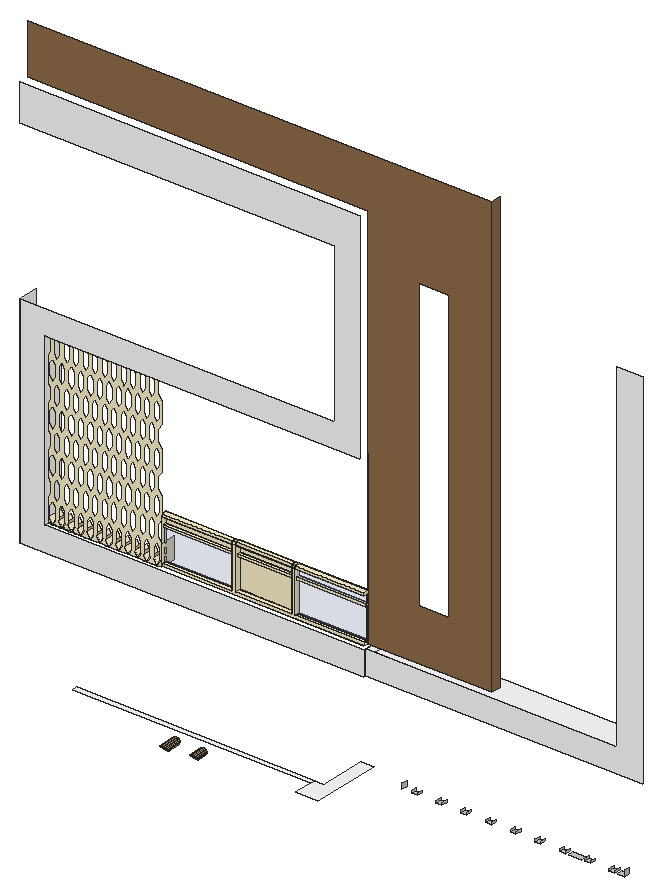
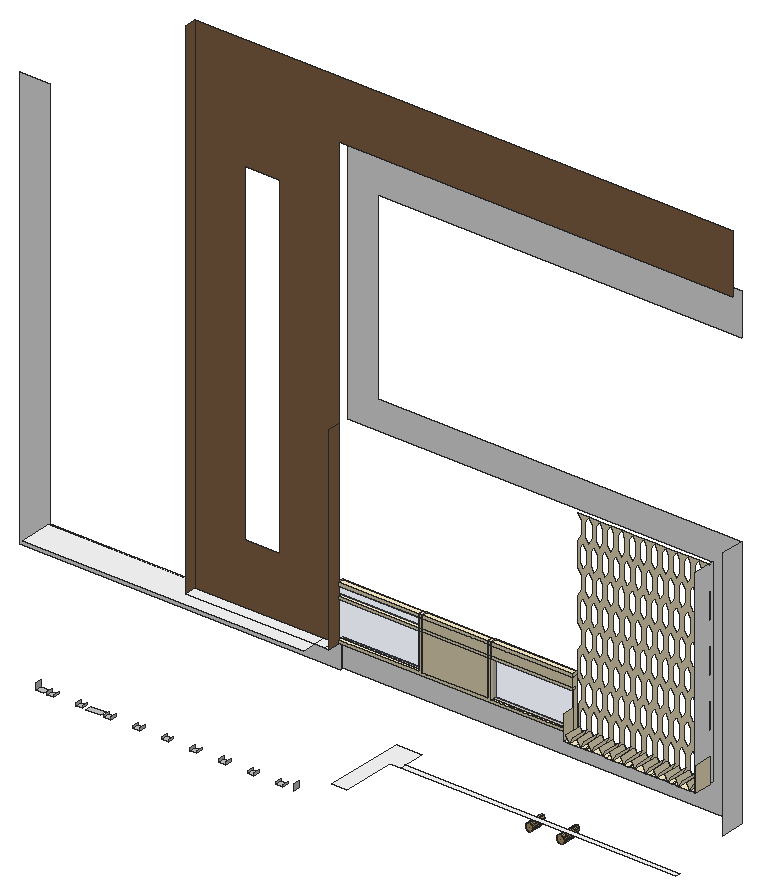
# SketchUp Ruby script. Lengths in inches.
U = 1.inch
M = Sketchup.active_model
def pt(a) = Geom::Point3d.new(a.map { |v| v * U })
def face(e, loops, mat)
  f = e.add_face(loops[0].map { |a| pt(a) })
  loops[1..].each { |l| e.add_face(l.map { |a| pt(a) }).erase! }
  f.material = f.back_material = mat if mat
  f
end
# faces: each face lists its corners as indices into pts; further lists are holes
def faces(e, pts, list, mat = nil) = list.each { |f| face(e, (f[0].is_a?(Array) ? f : [f]).map { |l| l.map { |i| pts[i] } }, mat) }
# xy, xz, yz: faces in a plane at the given z, y or x. An outline is a flat list of corners, or four numbers for a rectangle; further outlines are holes
def ring(l) = l.size == 4 ? [[l[0], l[1]], [l[2], l[1]], [l[2], l[3]], [l[0], l[3]]] : l.each_slice(2).to_a
def flat(e, list, mat, &to3) = list.each { |f| face(e, (f[0].is_a?(Array) ? f : [f]).map { |l| ring(l).map { |u, v| to3.(u, v) } }, mat) }
def xy(e, z, list, mat = nil) = flat(e, list, mat) { |x, y| [x, y, z] }
def xz(e, y, list, mat = nil) = flat(e, list, mat) { |x, z| [x, y, z] }
def yz(e, x, list, mat = nil) = flat(e, list, mat) { |y, z| [x, y, z] }
def lines(e, pts, list) = list.each { |a, b| e.add_line(pt(pts[a]), pt(pts[b])) }
# prism: a flat outline (further loops are holes) pulled along v
def prism(e, loops, v, mat = nil)
  f = face(e, loops, mat); d = Geom::Vector3d.new(v.map { |x| x * U })
  f.pushpull(f.normal.samedirection?(d) ? d.length : -d.length)
end
def box(e, o, s, mat = nil) = prism(e, [[o, [o[0] + s[0], o[1], o[2]], [o[0] + s[0], o[1] + s[1], o[2]], [o[0], o[1] + s[1], o[2]]]], [0, 0, s[2]], mat)
def at(x, y, z, deg = 0) = Geom::Transformation.translation(pt([x, y, z])) * Geom::Transformation.rotation(ORIGIN, Z_AXIS, deg.degrees)
def axes(o, x, y, z) = Geom::Transformation.new([*x, 0, *y, 0, *z, 0, *pt(o).to_a, 1])
def part(name) = M.definitions.add(name)
# library, detail: a bought-in or finely detailed component or shape, given as its bounding box
def library(name, o, s) = part(name).tap { |d| box(d.entities, o, s) }
def detail(e, o, s) = box(e.add_group.entities, o, s)
def put(e, d, t, mat = nil) = e.add_instance(d, t).tap { |i| i.material = mat if mat }
def group(e, t, mat = nil) = e.add_group.tap { |g| g.transformation = t; g.material = mat if mat }.entities
root = M.entities
M.materials.add("D01_Frost_White").color = [255, 242, 206]
M.materials.add("Glass_Sky Reflection_01").color = [126, 138, 183]
M.materials["Glass_Sky Reflection_01"].alpha = 0.25
M.materials.add("M00_Soft_Cloud").color = [255, 255, 255]
M.materials.add("Metal_Perforated_03_1K").color = [205, 205, 205]
M.materials.add("Plywood_08_1K").color = [202, 166, 113]
M.materials.add("Wood_Floor_01_1K").color = [146, 111, 76]
xy(root,51.6968,[[394.8388,115.4372,398.9652,119.1663],[412.2906,115.4372,416.417,119.1663],[429.7424,115.4372,433.8688,119.1663],[447.1942,115.4372,451.3206,119.1663],[464.646,115.4372,468.7724,119.1663],
  [482.0978,115.4372,486.2242,119.1663],[499.5496,115.4372,503.676,119.1663],[517.0014,115.4372,521.1278,119.1663],[534.4532,115.4372,538.5796,119.1663]],"Metal_Perforated_03_1K")
xy(root,51.7981,[[505.7245,115.4372,514.9529,119.1663],[540.6281,115.4372,545.2423,119.1663]],"Metal_Perforated_03_1K")
xy(root,60,[[353.5364,64.7712,369.0099,64.7712,369.0099,114,360.228,114,360.228,81.2712,353.5364,81.2712],[185.5364,78.2712,353.5364,81.2712]],"M00_Soft_Cloud")
xy(root,137.0192,[[209.933,109.0676,210.1614,119.6039],[210.1614,109.0676,211.0379,119.6039],[211.0379,109.0676,213.2784,119.6039],[213.2784,109.0676,216.6239,119.6039],[216.6239,109.0676,219.9694,119.6039],
  [219.9694,109.0676,223.3148,119.6039]],"D01_Frost_White")
xy(root,137.0192,[[368.5859,108.0124,368.7779,112.9098],[368.7779,108.0124,375,112.9098],[375,108.0124,546,108.0124,546,128.0311,375,128.0311,375,120,453.2434,120,453.2434,112.9098,375,112.9098],[366,112.9098,368.5859,120],[368.5859,112.9098,368.7779,120],
  [368.7779,112.9098,375,120],[368.7779,112.9098,375,120],[375,112.9098,453.2434,120]],"M00_Soft_Cloud")
xy(root,137.0253,[[183.1692,109.0676,183.3976,119.6039],[183.3976,109.0676,184.2742,119.6039],[184.2742,109.0676,186.5147,119.6039],[186.5147,109.0676,189.8602,119.6039],[189.8602,109.0676,193.2056,119.6039],
  [193.2056,109.0676,197.6561,119.6039],[197.6561,109.0676,199.8966,119.6039],[199.8966,109.0676,206.5875,119.6039],[206.5875,109.0676,209.933,119.6039]],"D01_Frost_White")
xy(root,137.0314,[[156.4055,109.0676,156.6339,119.6039],[156.6339,109.0676,157.5105,119.6039],[157.5105,109.0676,159.751,119.6039],[159.751,109.0676,163.0964,119.6039],[163.0964,109.0676,166.4419,119.6039],
  [166.4419,109.0676,169.7874,119.6039],[169.7874,109.0676,170.0158,119.6039],[170.0158,109.0676,170.8923,119.6039],[170.8923,109.0676,173.1328,119.6039],[173.1328,109.0676,179.8238,119.6039],
  [179.8238,109.0676,183.1692,119.6039]],"D01_Frost_White")
xy(root,137.0374,[[143.0236,109.0676,143.252,119.6039],[143.252,109.0676,144.1286,119.6039],[144.1286,109.0676,146.3691,119.6039],[146.3691,109.0676,153.06,119.6039],[153.06,109.0676,156.4055,119.6039]],"D01_Frost_White")
xy(root,137.5531,[[223.3148,109.5873,366.1463,113.1759]],"D01_Frost_White")
xy(root,139.4984,[[223.3148,109.5873,272.8822,111.884],[275.1001,109.5873,314.9232,113.1759],[317.1411,109.5873,366.1463,111.3816],[317.1411,111.3816,366.1463,113.1759],[223.3148,111.884,272.8822,113.1759]],"D01_Frost_White")
xy(root,161.637,[[223.3148,110.5921,366.1463,113.1759]],"D01_Frost_White")
xy(root,163.1544,[[223.3148,110.5921,366.1463,113.1759]],"D01_Frost_White")
xy(root,168.938,[[223.3148,109.5873,366.1463,113.1759]],"D01_Frost_White")
xy(root,170.8834,[[223.3148,109.5873,272.8822,113.1759],[272.8822,109.5873,275.1001,113.1759],[275.1001,109.5873,314.9232,113.1759],[314.9232,109.5873,317.1411,113.1759],[317.1411,109.5873,366.1463,113.1759]],"D01_Frost_White")
xz(root,78.2712,[[258.3445,50.6009,257.7234,50.6827,257.1447,50.9224,256.6477,51.3038,256.2664,51.8007,256.0266,52.3795,255.9449,53.0005,256.0266,53.6216,256.2664,54.2003,256.6477,54.6973,257.1447,55.0786,257.7234,55.3184,258.3445,55.4001,258.9655,55.3184,259.5443,55.0786,260.0412,54.6973,260.4226,54.2003,260.6623,53.6216,260.7441,53.0005,260.6623,52.3795,260.4226,51.8007,260.0412,51.3038,259.5443,50.9224,258.9655,50.6827],[277.4723,50.6009,276.8512,50.6827,276.2725,50.9224,275.7755,51.3038,275.3941,51.8007,275.1544,52.3795,275.0727,53.0005,275.1544,53.6216,275.3941,54.2003,275.7755,54.6973,276.2725,55.0786,276.8512,55.3184,277.4723,55.4001,278.0933,55.3184,278.6721,55.0786,279.169,54.6973,279.5504,54.2003,279.7901,53.6216,279.8719,53.0005,279.7901,52.3795,279.5504,51.8007,279.169,51.3038,278.6721,50.9224,278.0933,50.6827]],"Plywood_08_1K")
xz(root,105.8195,[[126,120,368.7779,120,368.7779,137.0192,143.4397,137.0192,143.4397,257.0192,366,257.0192,366,411.0577,126,411.0577,126,385.4776,348,385.4776,348,274.0384,126,274.0384]],"M00_Soft_Cloud")
xz(root,108.0124,[[368.5859,119.9631,564,119.9631,564,377.4389,546,377.4389,546,137.0192,368.5859,137.0192]],"M00_Soft_Cloud")
xz(root,109.0676,[[[209.933,137.0192,213.2784,137.0192,211.0744,140.7687,211.0744,148.2675,213.2784,152.0169,215.4825,148.2675,215.4825,140.7687,213.2784,137.0192,219.9694,137.0192,217.7653,140.7687,217.7653,148.2675,219.9694,152.0169,222.1734,148.2675,222.1734,140.7687,219.9694,137.0192,223.3148,137.0192,223.3148,152.0169,221.1108,155.7664,221.1108,163.2652,223.3148,167.0147,223.3148,182.0124,221.1108,185.7618,221.1108,193.2607,223.3148,197.0101,223.3077,197.0101,223.3077,212.0078,221.1037,215.7573,221.1037,223.2561,223.3077,227.0056,223.3077,242.0033,221.1037,245.7527,221.1037,253.2516,223.3077,257.001,216.6168,257.001,218.8208,253.2516,218.8208,245.7527,216.6168,242.0033,214.4127,245.7527,214.4127,253.2516,216.6168,257.001,209.933,257.001,209.933,256.9889,212.1299,253.2516,212.1299,245.7527,209.933,242.0154,209.933,242.0094,209.9312,242.0124,207.7289,245.7588,207.7289,253.2576,209.9276,256.998,209.9258,257.001,209.9294,257.001,209.933,257.0071,203.242,257.0071,205.4461,253.2576,205.4461,245.7588,203.242,242.0094,201.038,245.7588,201.038,253.2576,203.242,257.0071,196.5511,257.0071,196.5529,257.004,196.5547,257.004,196.5547,257.001,198.7552,253.2576,198.7552,245.7588,198.7444,245.7406,198.7409,245.7345,198.7337,245.7225,196.5404,242.0154,196.5368,242.0094,196.5261,242.0276,195.4366,243.8932,195.801,243.2733,194.3399,245.783,194.3399,245.7709,194.3363,245.777,194.3364,245.7891,194.3363,245.7892,194.3364,245.8134,194.3399,249.5264,194.3399,248.2868,194.347,253.2698,194.3542,253.2819,195.0829,254.5216,195.4473,255.1415,196.5422,257.004,189.8548,257.004,192.0571,253.2576,192.0571,245.7588,189.853,242.0094,187.649,245.7588,187.649,253.2576,189.8512,257.004,183.1639,257.004,185.3661,253.2576,185.3661,245.7588,183.1675,242.0185,183.1639,242.0124,183.1639,242.0245,180.9652,245.7649,180.9652,253.2637,183.1639,257.004,183.1621,257.0071,183.1657,257.0071,183.1692,257.0132,176.4783,257.0132,178.6824,253.2637,178.6824,245.7649,176.4783,242.0154,174.2743,245.7649,174.2743,253.2637,176.4783,257.0132,169.7874,257.0132,171.9878,253.2576,171.9843,245.7649,169.7802,242.0276,167.5797,245.7709,167.5797,253.2698,167.5833,253.2759,169.7838,257.0192,163.0929,257.0192,165.2969,253.2698,165.2969,245.7709,163.0929,242.0215,160.8888,245.7709,160.8888,253.2698,163.0929,257.0192,156.4055,257.0192,156.4037,257.0162,158.606,253.2698,158.606,245.7709,156.4037,242.0245,154.2015,245.7709,154.2015,253.2698,156.4037,257.0162,156.4019,257.0192,149.7146,257.0192,151.9186,253.2698,151.9186,245.7709,149.7146,242.0215,147.5105,245.7709,147.5105,253.2698,149.7146,257.0192,143.0236,257.0192,145.2277,253.2698,145.2277,245.7709,143.0236,242.0215,143.0236,227.0238,145.2277,223.2743,145.2277,215.7755,143.0236,212.0261,143.0236,197.0283,143.0271,197.0224,143.0272,197.0223,145.2277,193.2789,145.2277,185.78,143.0236,182.0306,143.0236,167.0329,145.2277,163.2835,145.2277,155.7846,143.0236,152.0352,143.0236,137.0374,146.3691,137.0374,144.165,140.7869,144.165,148.2857,146.3691,152.0352,148.5731,148.2857,148.5731,140.7869,146.3691,137.0374,153.06,137.0374,150.856,140.7869,150.856,148.2857,153.06,152.0352,155.2641,148.2857,155.2641,140.7869,153.06,137.0374,156.4055,137.0374,156.4055,137.0314,159.751,137.0314,157.5469,140.7808,157.5469,148.2797,159.751,152.0291,161.955,148.2797,161.955,140.7808,159.751,137.0314,166.4419,137.0314,164.2379,140.7808,164.2379,148.2797,166.4419,152.0291,168.6459,148.2797,168.6459,140.7808,166.4419,137.0314,173.1328,137.0314,170.9288,140.7808,170.9288,148.2797,173.1328,152.0291,175.3369,148.2797,175.3369,140.7808,173.1328,137.0314,179.8238,137.0314,177.6197,140.7808,177.6197,148.2797,179.8238,152.0291,182.0278,148.2797,182.0278,140.7808,179.8238,137.0314,183.1692,137.0314,183.1692,137.0253,186.5147,137.0253,184.3107,140.7747,184.3107,148.2736,186.5147,152.023,188.7188,148.2736,188.7188,140.7747,186.5147,137.0253,193.2056,137.0253,191.0016,140.7747,191.0016,148.2736,193.2056,152.023,195.4097,148.2736,195.4097,140.7747,193.2056,137.0253,199.8966,137.0253,197.6925,140.7747,197.6925,148.2736,199.8966,152.023,202.1006,148.2736,202.1006,140.7747,199.8966,137.0253,206.5875,137.0253,204.3835,140.7747,204.3835,148.2736,206.5875,152.023,208.7916,148.2736,208.7916,140.7747,206.5875,137.0253,209.933,137.0253],[169.7874,182.0245,168.6907,183.8901,167.5869,185.7557,167.5869,185.7679,167.5833,185.774,167.5833,189.5052,167.5797,193.2546,167.5833,193.2607,167.5833,193.2728,168.68,195.1384,169.7802,197.0223,169.7874,197.0223,169.7909,197.0163,169.7909,197.0162,170.884,195.1567,171.9878,193.2911,171.9879,193.2789,171.9914,193.2728,171.9914,189.5416,171.995,185.7922,171.9914,185.7861,171.9914,185.774,170.8947,183.9084,169.7945,182.0245,169.7909,182.0306],[189.8602,182.0185,187.6561,185.7679,187.6561,193.2668,189.8566,197.0101,189.8495,197.0101,189.8514,197.0134,189.853,197.0162,189.8602,197.0162,189.8637,197.0101,192.0642,193.2668,192.0642,185.7679],[196.5511,182.0185,194.3471,185.7679,194.3471,193.2668,196.5475,197.0101,196.5404,197.0101,196.544,197.0162,196.5511,197.0162,196.5546,197.0102,196.5547,197.0101,198.7552,193.2668,198.7552,185.7679],[216.6239,182.0124,214.4199,185.7618,214.4199,193.2607,216.6203,197.004,216.6184,197.0073,216.6168,197.0101,216.6239,197.0101,218.828,193.2607,218.828,185.7618],[163.0964,182.0245,160.8924,185.774,160.8924,193.2728,163.0964,197.0223,163.0893,197.0223,163.0912,197.0256,163.0929,197.0283,163.0945,197.0256,163.0964,197.0223,165.3005,193.2728,165.3005,185.774],[209.933,182.0124,209.933,182.0185,207.7289,185.7679,207.7289,193.2668,209.9276,197.0071,209.9258,197.0101,209.9294,197.0101,209.933,197.0162,209.933,197.0101,212.137,193.2607,212.137,185.7618],[203.242,212.0139,201.038,215.7633,201.038,223.2622,203.242,227.0116,205.4461,223.2622,205.4461,215.7633],[163.0929,212.0261,160.8888,215.7755,160.8888,223.2743,163.0929,227.0238,165.2969,223.2743,165.2969,215.7755],[189.853,212.0139,187.649,215.7633,187.649,223.2622,189.853,227.0116,192.0571,223.2622,192.0571,215.7633],[216.6168,212.0078,214.4127,215.7573,214.4127,223.2561,216.6168,227.0056,218.8208,223.2561,218.8208,215.7573],[196.544,212.0139,194.3399,215.7633,194.3399,223.2622,196.544,227.0116,198.748,223.2622,198.748,215.7633],[206.5875,197.0162,204.3835,200.7656,204.3835,208.2645,206.5875,212.0139,208.7916,208.2645,208.7916,200.7656],[199.8966,197.0162,197.6925,200.7656,197.6925,208.2645,199.8966,212.0139,202.1006,208.2645,202.1006,200.7656],[186.5076,197.0162,184.3035,200.7656,184.3035,208.2645,186.5076,212.0139,188.7116,208.2645,188.7116,200.7656],[166.4383,197.0283,164.2343,200.7778,164.2343,208.2766,166.4383,212.0261,168.6424,208.2766,168.6424,200.7778],[159.7474,197.0283,157.5433,200.7778,157.5433,208.2766,159.7474,212.0261,161.9514,208.2766,161.9514,200.7778],[193.1985,197.0162,190.9945,200.7656,190.9945,208.2645,193.1985,212.0139,195.4025,208.2645,195.4025,200.7656],[219.9622,197.0101,217.7582,200.7595,217.7582,208.2584,219.9622,212.0078,222.1663,208.2584,222.1663,200.7595],[213.2713,197.0101,211.0673,200.7595,211.0673,208.2584,213.2713,212.0078,215.4754,208.2584,215.4754,200.7595],[189.8602,152.023,187.6561,155.7725,187.6561,163.2713,189.8602,167.0207,192.0642,163.2713,192.0642,155.7725],[176.4783,212.02,174.2743,215.7694,174.2743,223.2683,176.4783,227.0177,178.6824,223.2683,178.6824,215.7694],[156.4055,182.0245,156.4055,182.0306,154.2015,185.78,154.2015,193.2789,156.4019,197.0223,156.4055,197.0283,156.4055,197.0223,158.6095,193.2728,158.6095,185.774],[149.7146,212.0261,147.5105,215.7755,147.5105,223.2743,149.7146,227.0238,151.9186,223.2743,151.9186,215.7755],[163.0964,152.0291,160.8924,155.7785,160.8924,163.2774,163.0964,167.0268,165.3005,163.2774,165.3005,155.7785],[176.4783,182.0245,174.2743,185.774,174.2743,193.2728,176.4747,197.0162,176.4767,197.0195,176.4783,197.0223,176.4799,197.0195,176.4819,197.0162,178.6824,193.2728,178.6824,185.774],[149.7146,152.0352,147.5105,155.7846,147.5105,163.2835,149.7146,167.0329,151.9186,163.2835,151.9186,155.7846],[156.4055,152.0291,156.4055,152.0352,154.2015,155.7846,154.2015,163.2835,156.4055,167.0329,156.4055,167.0268,158.6095,163.2774,158.6095,155.7785],[149.7146,182.0306,147.5105,185.78,147.5105,193.2789,149.711,197.0223,149.7129,197.0256,149.7146,197.0283,149.7162,197.0256,149.7181,197.0223,151.9186,193.2789,151.9186,185.78],[169.7874,152.0291,167.5833,155.7785,167.5833,163.2774,169.7874,167.0268,171.9914,163.2774,171.9914,155.7785],[183.1692,152.023,183.1692,152.0291,180.9652,155.7785,180.9652,163.2774,183.1692,167.0268,183.1692,167.0207,185.3733,163.2713,185.3733,155.7725],[179.8238,197.0223,177.6197,200.7717,177.6197,208.2706,179.8238,212.02,182.0278,208.2706,182.0278,200.7717],[173.1328,197.0223,170.9288,200.7717,170.9288,208.2706,173.1328,212.02,175.3369,208.2706,175.3369,200.7717],[146.3691,197.0283,144.165,200.7778,144.165,208.2766,146.3691,212.0261,148.5731,208.2766,148.5731,200.7778],[153.06,197.0283,150.856,200.7778,150.856,208.2766,153.06,212.0261,155.2641,208.2766,155.2641,200.7778],[196.5511,152.023,194.3471,155.7725,194.3471,163.2713,196.5511,167.0207,198.7552,163.2713,198.7552,155.7725],[176.4783,152.0291,174.2743,155.7785,174.2743,163.2774,176.4783,167.0268,178.6824,163.2774,178.6824,155.7785],[179.8238,167.0268,177.6197,170.7762,177.6197,178.2751,179.8238,182.0245,182.0278,178.2751,182.0278,170.7762],[216.6239,152.0169,214.4199,155.7664,214.4199,163.2652,216.6239,167.0147,218.828,163.2652,218.828,155.7664],[173.1328,167.0268,170.9288,170.7762,170.9288,178.2751,173.1328,182.0245,175.3369,178.2751,175.3369,170.7762],[153.06,167.0329,150.856,170.7823,150.856,178.2812,153.06,182.0306,155.2641,178.2812,155.2641,170.7823],[209.933,152.0169,209.933,152.023,207.7289,155.7725,207.7289,163.2713,209.933,167.0207,209.933,167.0147,212.137,163.2652,212.137,155.7664],[146.3691,167.0329,144.165,170.7823,144.165,178.2812,146.3691,182.0306,148.5731,178.2812,148.5731,170.7823],[186.5147,167.0207,184.3107,170.7702,184.3107,178.269,186.5147,182.0185,188.7188,178.269,188.7188,170.7702],[193.2056,167.0207,191.0016,170.7702,191.0016,178.269,193.2056,182.0185,195.4097,178.269,195.4097,170.7702],[173.1328,227.0177,170.9288,230.7671,170.9288,238.266,173.1328,242.0154,175.3369,238.266,175.3369,230.7671],[179.8238,227.0177,177.6197,230.7671,177.6197,238.266,179.8238,242.0154,182.0278,238.266,182.0278,230.7671],[166.4419,167.0268,164.2379,170.7762,164.2379,178.2751,166.4419,182.0245,168.6459,178.2751,168.6459,170.7762],[159.751,167.0268,157.5469,170.7762,157.5469,178.2751,159.751,182.0245,161.955,178.2751,161.955,170.7762],[203.242,182.0185,201.038,185.7679,201.038,193.2668,203.2385,197.0101,203.2404,197.0134,203.242,197.0162,203.2437,197.0134,203.2456,197.0101,205.4461,193.2668,205.4461,185.7679],[153.06,227.0238,150.856,230.7732,150.856,238.2721,153.06,242.0215,155.2641,238.2721,155.2641,230.7732],[146.3691,227.0238,144.165,230.7732,144.165,238.2721,146.3691,242.0215,148.5731,238.2721,148.5731,230.7732],[203.242,152.023,201.038,155.7725,201.038,163.2713,203.242,167.0207,205.4461,163.2713,205.4461,155.7725],[193.1985,227.0116,190.9945,230.7611,190.9945,238.2599,193.1985,242.0094,195.4025,238.2599,195.4025,230.7611],[199.8966,227.0116,197.6925,230.7611,197.6925,238.2599,199.8966,242.0094,202.1006,238.2599,202.1006,230.7611],[206.5875,227.0116,204.3835,230.7611,204.3835,238.2599,206.5875,242.0094,208.7916,238.2599,208.7916,230.7611],[159.7474,227.0238,157.5433,230.7732,157.5433,238.2721,159.7474,242.0215,161.9514,238.2721,161.9514,230.7732],[166.4383,227.0238,164.2343,230.7732,164.2343,238.2721,166.4383,242.0215,168.6424,238.2721,168.6424,230.7732],[186.5076,227.0116,184.3035,230.7611,184.3035,238.2599,186.5076,242.0094,188.7116,238.2599,188.7116,230.7611],[213.2713,227.0056,211.0673,230.755,211.0673,238.2539,213.2713,242.0033,215.4754,238.2539,215.4754,230.755],[219.9622,227.0056,217.7582,230.755,217.7582,238.2539,219.9622,242.0033,222.1663,238.2539,222.1663,230.755],[206.5875,167.0207,204.3835,170.7702,204.3835,178.269,206.5875,182.0185,208.7916,178.269,208.7916,170.7702],[199.8966,167.0207,197.6925,170.7702,197.6925,178.269,199.8966,182.0185,202.1006,178.269,202.1006,170.7702],[213.2784,167.0147,211.0744,170.7641,211.0744,178.263,213.2784,182.0124,215.4825,178.263,215.4825,170.7641],[219.9694,167.0147,217.7653,170.7641,217.7653,178.263,219.9694,182.0124,222.1734,178.263,222.1734,170.7641],[183.1692,182.0185,183.1692,182.0245,180.9652,185.774,180.9652,193.2728,183.1639,197.0132,183.1656,197.0102,183.1657,197.0101,183.1728,197.0101,185.3733,193.2668,185.3733,185.7679],[169.7802,212.0321,167.5797,215.7755,167.5797,223.2743,167.5833,223.2804,169.7874,227.0177,171.9878,223.2622,171.9843,215.7694],[156.4037,212.0291,154.2015,215.7755,154.2015,223.2743,156.4037,227.0207,158.606,223.2743,158.606,215.7755],[209.933,212.0139,209.9312,212.0169,207.7289,215.7633,207.7289,223.2622,209.9276,227.0025,209.933,227.0116,209.933,226.9934,212.1299,223.2561,212.1299,215.7573,209.933,212.02],[183.1639,212.0169,183.1639,212.0291,180.9652,215.7694,180.9652,223.2683,183.1639,227.0086,185.3661,223.2622,185.3661,215.7633,183.1675,212.023],[195.4366,243.8932,194.3399,245.7588,194.3399,245.7709],[194.3399,249.5264,194.3399,253.2576,194.3435,253.2637]],[156.4091,137.0253,159.751,137.0253,159.751,137.0303,157.5105,137.0314,156.6339,137.0314,156.409,137.0254],[159.751,137.0253,163.0929,137.0253,163.0948,137.0286,159.751,137.0303],[169.7838,137.0253,169.7874,137.0314,166.4419,137.0314,166.4419,137.027],[156.409,137.0254,156.6339,137.0314,156.4055,137.0314],
  [163.0948,137.0286,163.0981,137.0286,163.0964,137.0314],[159.751,137.0303,159.751,137.0314,157.5105,137.0314],[143.0236,137.0314,143.252,137.0374,143.0236,137.0374],[143.0236,137.0314,146.3691,137.0314,146.3691,137.0363,144.1286,137.0374,143.252,137.0374],[146.3691,137.0314,153.06,137.0314,153.06,137.033,146.3691,137.0363],
  [156.4055,137.0314,156.4055,137.0374,153.06,137.0374,153.06,137.033],[153.06,137.033,153.06,137.0374,146.3691,137.0374,146.3691,137.0363],[146.3691,137.0363,146.3691,137.0374,144.1286,137.0374]],"D01_Frost_White")
xz(root,109.5873,[[223.3148,137.5531,366.1463,137.5531,366.1463,139.4984,317.1411,139.4984,317.1411,168.938,314.9232,168.938,314.9232,139.4984,275.1001,139.4984,275.1001,168.938,272.8822,168.938,272.8822,139.4984,223.3148,139.4984],[223.3148,168.938,272.8822,170.8834],[272.8822,168.938,275.1001,170.8834],[275.1001,168.938,314.9232,170.8834],[314.9232,168.938,317.1411,170.8834],
  [317.1411,168.938,366.1463,170.8834]],"D01_Frost_White")
xz(root,110.5921,[[223.3148,161.637,366.1463,163.1544]],"D01_Frost_White")
xz(root,111.3816,[[317.1411,139.4984,366.1463,168.938]],"Glass_Sky Reflection_01")
xz(root,111.884,[[223.3148,139.4984,272.8822,161.637]],"Glass_Sky Reflection_01")
xz(root,112.9098,[[[366,137.0192,453.2434,137.0192,453.2434,447.0577,126,447.0577,126,411.0577,366,411.0577],[402.037,173.8079,423.1418,377.6765]]],"Wood_Floor_01_1K")
xz(root,113.1759,[[223.3148,137.5531,223.3148,139.4984,272.8822,139.4984,272.8822,161.637,275.1001,161.637,275.1001,139.4984,314.9232,139.4984,314.9232,161.637,317.1411,161.637,317.1411,139.4984,366.1463,139.4984,366.1463,137.5531],[275.1001,139.4984,314.9232,161.637],[223.3148,161.637,272.8822,163.1544],[272.8822,161.637,275.1001,163.1544],[275.1001,161.637,314.9232,163.1544],
  [314.9232,161.637,317.1411,163.1544],[317.1411,161.637,366.1463,163.1544],[223.3148,163.1544,272.8822,168.938],[272.8822,163.1544,275.1001,168.938],[275.1001,163.1544,314.9232,168.938],
  [314.9232,163.1544,317.1411,168.938],[223.3148,168.938,272.8822,170.8834],[272.8822,168.938,275.1001,170.8834],[275.1001,168.938,314.9232,170.8834],[314.9232,168.938,317.1411,170.8834],
  [317.1411,168.938,366.1463,170.8834]],"D01_Frost_White")
yz(root,126,[[105.8195,120,120,274.0384]],"M00_Soft_Cloud")
yz(root,143.0236,[[109.0676,137.0374,119.6039,152.0352]],"D01_Frost_White")
yz(root,143.4397,[[105.8195,137.0192,120,257.0192]],"M00_Soft_Cloud")
yz(root,156.4055,[[109.0676,137.0314,119.6039,137.0374]],"D01_Frost_White")
yz(root,183.1692,[[109.0676,137.0253,119.6039,137.0314]],"D01_Frost_White")
yz(root,209.933,[[109.0676,137.0192,119.6039,137.0253]],"D01_Frost_White")
yz(root,223.3148,[[109.0676,137.0192,119.6039,152.0169],[109.5873,137.0192,113.1759,137.5531],[109.5873,137.5531,113.1759,139.4984],[109.5873,139.4984,109.5873,168.938,113.1759,168.938,113.1759,163.1544,110.5921,163.1544,110.5921,161.637,111.884,161.637,111.884,139.4984],[111.884,139.4984,113.1759,161.637],
  [110.5921,161.637,113.1759,163.1544],[109.5873,168.938,113.1759,170.8834]],"D01_Frost_White")
yz(root,272.8822,[[109.5873,139.4984,113.1759,170.8834]],"D01_Frost_White")
yz(root,275.1001,[[109.5873,139.4984,113.1759,170.8834]],"D01_Frost_White")
yz(root,314.9232,[[109.5873,139.4984,113.1759,170.8834]],"D01_Frost_White")
yz(root,317.1411,[[109.5873,139.4984,113.1759,170.8834]],"D01_Frost_White")
yz(root,366,[[112.9098,137.0192,120,257.0192]],"Wood_Floor_01_1K")
yz(root,366.1463,[[110.5921,161.637,111.3816,163.1544],[111.3816,161.637,113.1759,163.1544],[109.5873,168.938,113.1759,170.8834]],"D01_Frost_White")
yz(root,388.1761,[[115.4372,51.7981,119.1663,55.6219]],"Metal_Perforated_03_1K")
yz(root,394.8388,[[115.4372,51.6968,119.1663,53.0313]],"Metal_Perforated_03_1K")
yz(root,398.9652,[[115.4372,51.6968,119.1663,53.0313]],"Metal_Perforated_03_1K")
yz(root,412.2906,[[115.4372,51.6968,119.1663,53.0313]],"Metal_Perforated_03_1K")
yz(root,416.417,[[115.4372,51.6968,119.1663,53.0313]],"Metal_Perforated_03_1K")
yz(root,429.7424,[[115.4372,51.6968,119.1663,53.0313]],"Metal_Perforated_03_1K")
yz(root,433.8688,[[115.4372,51.6968,119.1663,53.0313]],"Metal_Perforated_03_1K")
yz(root,447.1942,[[115.4372,51.6968,119.1663,53.0313]],"Metal_Perforated_03_1K")
yz(root,451.3206,[[115.4372,51.6968,119.1663,53.0313]],"Metal_Perforated_03_1K")
yz(root,453.2434,[[112.9098,137.0192,120,447.0577]],"Wood_Floor_01_1K")
yz(root,464.646,[[115.4372,51.6968,119.1663,53.0313]],"Metal_Perforated_03_1K")
yz(root,468.7724,[[115.4372,51.6968,119.1663,53.0313]],"Metal_Perforated_03_1K")
yz(root,482.0978,[[115.4372,51.6968,119.1663,53.0313]],"Metal_Perforated_03_1K")
yz(root,486.2242,[[115.4372,51.6968,119.1663,53.0313]],"Metal_Perforated_03_1K")
yz(root,499.5496,[[115.4372,51.6968,119.1663,53.0313]],"Metal_Perforated_03_1K")
yz(root,503.676,[[115.4372,51.6968,119.1663,53.0313]],"Metal_Perforated_03_1K")
yz(root,517.0014,[[115.4372,51.6968,119.1663,53.0313]],"Metal_Perforated_03_1K")
yz(root,521.1278,[[115.4372,51.6968,119.1663,53.0313]],"Metal_Perforated_03_1K")
yz(root,534.4532,[[115.4372,51.6968,119.1663,53.0313]],"Metal_Perforated_03_1K")
yz(root,538.5796,[[115.4372,51.6968,119.1663,53.0313]],"Metal_Perforated_03_1K")
yz(root,545.2423,[[115.4372,51.7981,119.1663,55.6219]],"Metal_Perforated_03_1K")
p = [[257.7234,78.2712,50.6827],[258.3445,78.2712,50.6009],[258.3445,70.3613,50.6009],[257.7234,70.2796,50.6827],[258.9655,78.2712,50.6827],[258.9655,70.2796,50.6827],
  [276.8512,78.2712,50.6827],[277.4723,78.2712,50.6009],[277.4723,72.8217,50.6009],[276.8512,72.7399,50.6827],[278.0933,78.2712,50.6827],[278.0933,72.7399,50.6827],
  [257.1447,78.2712,50.9224],[257.1447,70.0399,50.9224],[259.5443,78.2712,50.9224],[259.5443,70.0399,50.9224],[276.2725,78.2712,50.9224],[276.2725,72.5002,50.9224],
  [278.6721,78.2712,50.9224],[278.6721,72.5002,50.9224],[256.6477,78.2712,51.3038],[256.6477,69.6585,51.3038],[260.0412,78.2712,51.3038],[260.0412,69.6585,51.3038],
  [275.7755,78.2712,51.3038],[275.7755,72.1189,51.3038],[279.169,78.2712,51.3038],[279.169,72.1189,51.3038],[256.2664,78.2712,51.8007],[256.2664,69.1615,51.8007],
  [260.4226,78.2712,51.8007],[260.4226,69.1615,51.8007],[275.3941,78.2712,51.8007],[275.3941,71.6219,51.8007],[279.5504,78.2712,51.8007],[279.5504,71.6219,51.8007],
  [256.0266,78.2712,52.3795],[256.0266,68.5828,52.3795],[260.6623,78.2712,52.3795],[260.6623,68.5828,52.3795],[275.1544,78.2712,52.3795],[275.1544,71.0432,52.3795],
  [279.7901,78.2712,52.3795],[279.7901,71.0432,52.3795],[255.9449,78.2712,53.0005],[255.9449,67.9617,53.0005],[260.7441,78.2712,53.0005],[260.7441,67.9617,53.0005],
  [275.0727,78.2712,53.0005],[275.0727,70.4221,53.0005],[279.8719,78.2712,53.0005],[279.8719,70.4221,53.0005],[256.0266,78.2712,53.6216],[256.0266,67.3407,53.6216],
  [260.6623,78.2712,53.6216],[260.6623,67.3407,53.6216],[275.1544,78.2712,53.6216],[275.1544,69.801,53.6216],[279.7901,78.2712,53.6216],[279.7901,69.801,53.6216],
  [256.2664,78.2712,54.2003],[256.2664,66.7619,54.2003],[260.4226,78.2712,54.2003],[260.4226,66.7619,54.2003],[275.3941,78.2712,54.2003],[275.3941,69.2223,54.2003],
  [279.5504,78.2712,54.2003],[279.5504,69.2223,54.2003],[256.6477,78.2712,54.6973],[256.6477,66.265,54.6973],[260.0412,78.2712,54.6973],[260.0412,66.265,54.6973],
  [275.7755,78.2712,54.6973],[275.7755,68.7253,54.6973],[279.169,78.2712,54.6973],[279.169,68.7253,54.6973],[257.1447,78.2712,55.0786],[257.1447,65.8836,55.0786],
  [259.5443,78.2712,55.0786],[259.5443,65.8836,55.0786],[276.2725,78.2712,55.0786],[276.2725,68.344,55.0786],[278.6721,78.2712,55.0786],[278.6721,68.344,55.0786],
  [257.7234,78.2712,55.3184],[257.7234,65.6439,55.3184],[258.9655,78.2712,55.3184],[258.9655,65.6439,55.3184],[276.8512,78.2712,55.3184],[276.8512,68.1043,55.3184],
  [278.0933,78.2712,55.3184],[278.0933,68.1043,55.3184],[258.3445,78.2712,55.4001],[258.3445,65.5622,55.4001],[277.4723,78.2712,55.4001],[277.4723,68.0225,55.4001],
  [146.3691,109.0676,137.0374],[144.165,109.0676,140.7869],[144.165,119.6039,140.7869],[146.3691,119.6039,137.0374],[148.5731,109.0676,140.7869],[148.5731,119.6039,140.7869],
  [153.06,109.0676,137.0374],[150.856,109.0676,140.7869],[150.856,119.6039,140.7869],[153.06,119.6039,137.0374],[155.2641,109.0676,140.7869],[155.2641,119.6039,140.7869],
  [159.751,109.0676,137.0314],[157.5469,109.0676,140.7808],[157.5469,119.6039,140.7808],[159.751,119.6039,137.0314],[161.955,109.0676,140.7808],[161.955,119.6039,140.7808],
  [166.4419,109.0676,137.0314],[164.2379,109.0676,140.7808],[164.2379,119.6039,140.7808],[166.4419,119.6039,137.0314],[168.6459,109.0676,140.7808],[168.6459,119.6039,140.7808],
  [173.1328,109.0676,137.0314],[170.9288,109.0676,140.7808],[170.9288,119.6039,140.7808],[173.1328,119.6039,137.0314],[175.3369,109.0676,140.7808],[175.3369,119.6039,140.7808],
  [179.8238,109.0676,137.0314],[177.6197,109.0676,140.7808],[177.6197,119.6039,140.7808],[179.8238,119.6039,137.0314],[182.0278,109.0676,140.7808],[182.0278,119.6039,140.7808],
  [186.5147,109.0676,137.0253],[184.3107,109.0676,140.7747],[184.3107,119.6039,140.7747],[186.5147,119.6039,137.0253],[188.7188,109.0676,140.7747],[188.7188,119.6039,140.7747],
  [193.2056,109.0676,137.0253],[191.0016,109.0676,140.7747],[191.0016,119.6039,140.7747],[193.2056,119.6039,137.0253],[195.4097,109.0676,140.7747],[195.4097,119.6039,140.7747],
  [199.8966,109.0676,137.0253],[197.6925,109.0676,140.7747],[197.6925,119.6039,140.7747],[199.8966,119.6039,137.0253],[202.1006,109.0676,140.7747],[202.1006,119.6039,140.7747],
  [206.5875,109.0676,137.0253],[204.3835,109.0676,140.7747],[204.3835,119.6039,140.7747],[206.5875,119.6039,137.0253],[208.7916,109.0676,140.7747],[208.7916,119.6039,140.7747],
  [213.2784,109.0676,137.0192],[211.0744,109.0676,140.7687],[211.0744,119.6039,140.7687],[213.2784,119.6039,137.0192],[215.4825,109.0676,140.7687],[215.4825,119.6039,140.7687],
  [219.9694,109.0676,137.0192],[217.7653,109.0676,140.7687],[217.7653,119.6039,140.7687],[219.9694,119.6039,137.0192],[222.1734,109.0676,140.7687],[222.1734,119.6039,140.7687],
  [258.3445,78.2712,53.0005],[258.3445,67.9617,53.0005],[277.4723,78.2712,53.0005],[277.4723,70.4221,53.0005],[153.06,109.0676,137.0314],[156.4055,109.0676,137.0314],
  [156.4055,109.0676,137.0253],[156.409,109.0676,137.0254],[163.0981,109.0676,137.0286],[166.4419,109.0676,137.027],[156.4091,109.0676,137.0253],[166.4419,109.0676,137.0253],
  [169.7838,109.0676,137.0253],[163.0929,109.0676,137.0253],[163.1,109.0676,137.0253],[169.7874,109.0676,137.0253],[169.7874,109.0676,137.0314]]
faces(root,p,[[0,1,2,3],[1,4,5,2],[6,7,8,9],[7,10,11,8],[12,0,3,13],[4,14,15,5],[16,6,9,17],[10,18,19,11],
  [20,12,13,21],[14,22,23,15],[24,16,17,25],[18,26,27,19],[28,20,21,29],[22,30,31,23],[32,24,25,33],[26,34,35,27],
  [36,28,29,37],[30,38,39,31],[40,32,33,41],[34,42,43,35],[44,36,37,45],[38,46,47,39],[48,40,41,49],[42,50,51,43],
  [52,44,45,53],[46,54,55,47],[56,48,49,57],[50,58,59,51],[60,52,53,61],[54,62,63,55],[64,56,57,65],[58,66,67,59],
  [68,60,61,69],[62,70,71,63],[72,64,65,73],[66,74,75,67],[76,68,69,77],[70,78,79,71],[80,72,73,81],[74,82,83,75],
  [84,76,77,85],[78,86,87,79],[88,80,81,89],[82,90,91,83],[92,84,85,93],[86,92,93,87],[94,88,89,95],[90,94,95,91]],"Plywood_08_1K")
faces(root,p,[[96,97,98,99],[100,96,99,101],[102,103,104,105],[106,102,105,107],[108,109,110,111],[112,108,111,113],[114,115,116,117],[118,114,117,119],
  [120,121,122,123],[124,120,123,125],[126,127,128,129],[130,126,129,131],[132,133,134,135],[136,132,135,137],[138,139,140,141],[142,138,141,143],
  [144,145,146,147],[148,144,147,149],[150,151,152,153],[154,150,153,155],[156,157,158,159],[160,156,159,161],[162,163,164,165],[166,162,165,167]],"D01_Frost_White")
lines(root,p,[[168,169],[170,171],[172,173],[174,175],[176,177],[174,178],[179,180],[173,174],[181,182],[183,184],[180,183],[182,179],
  [177,179]])
